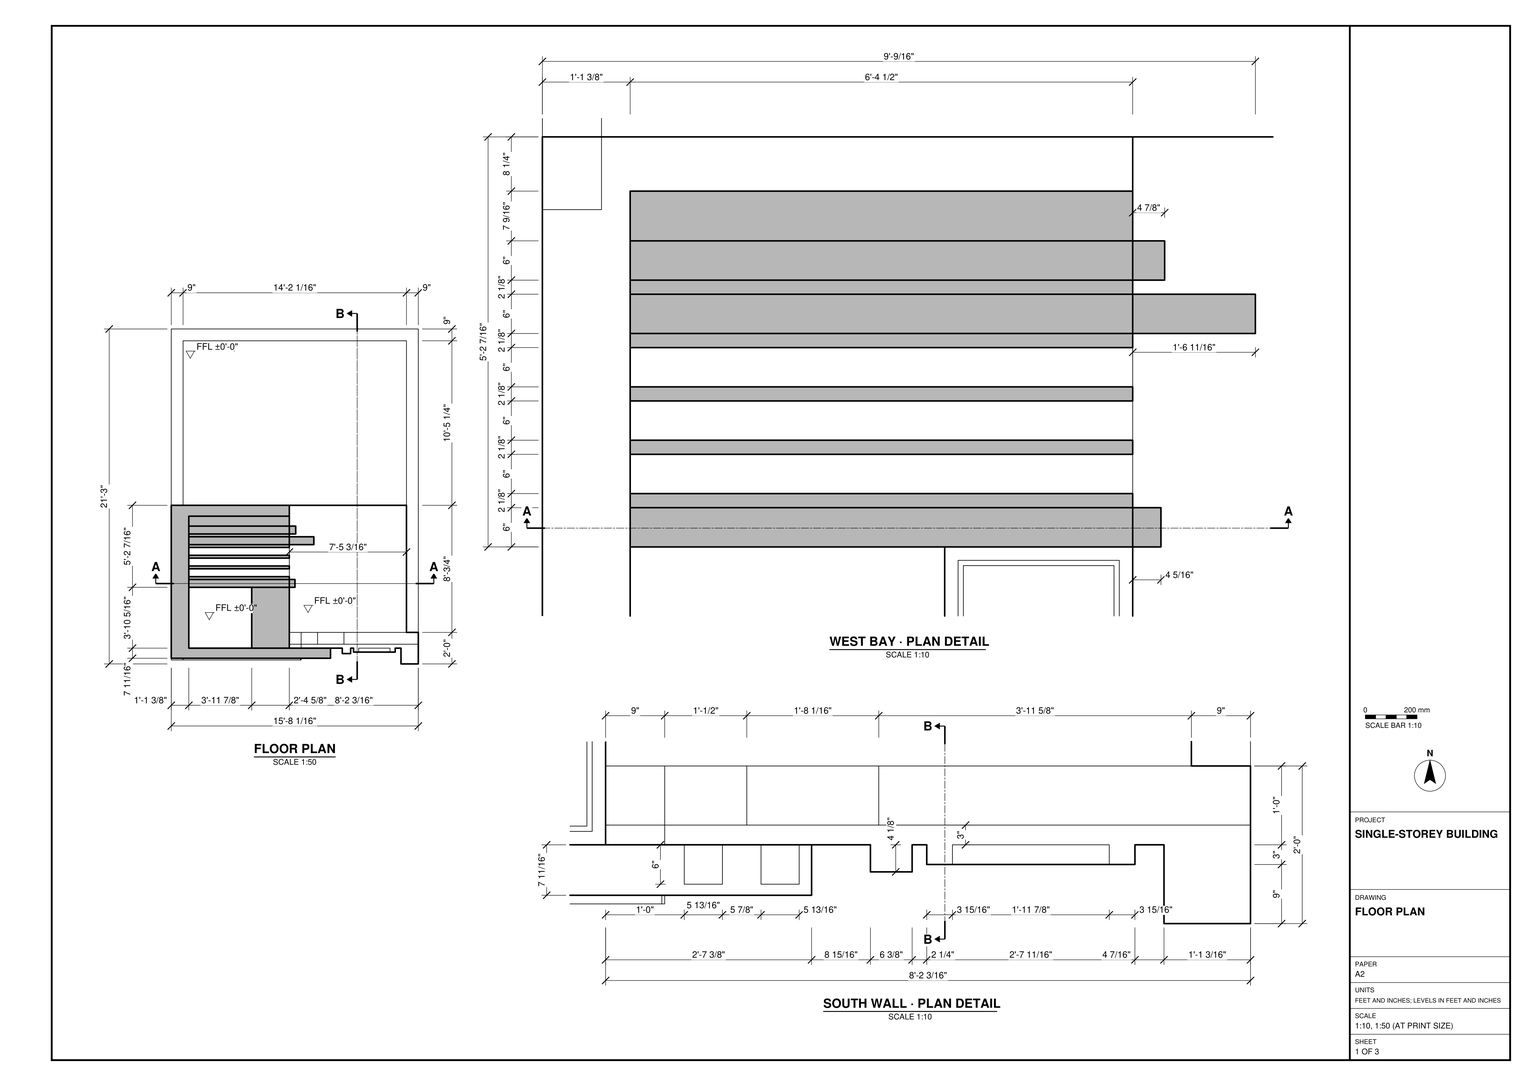
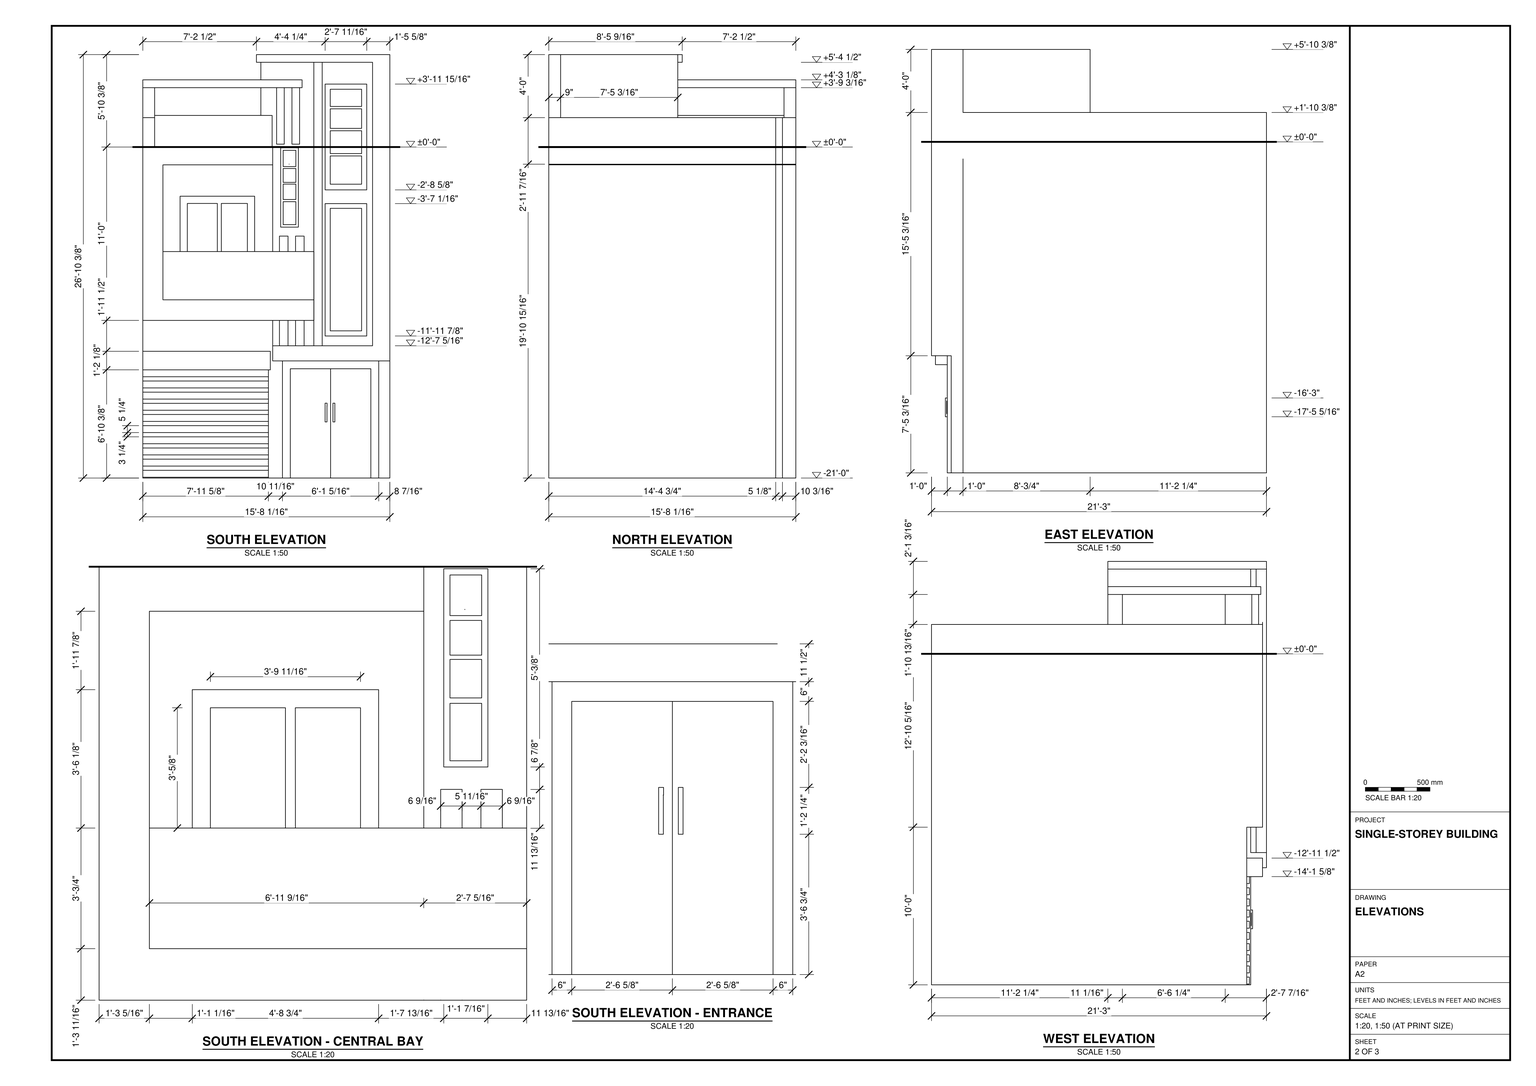
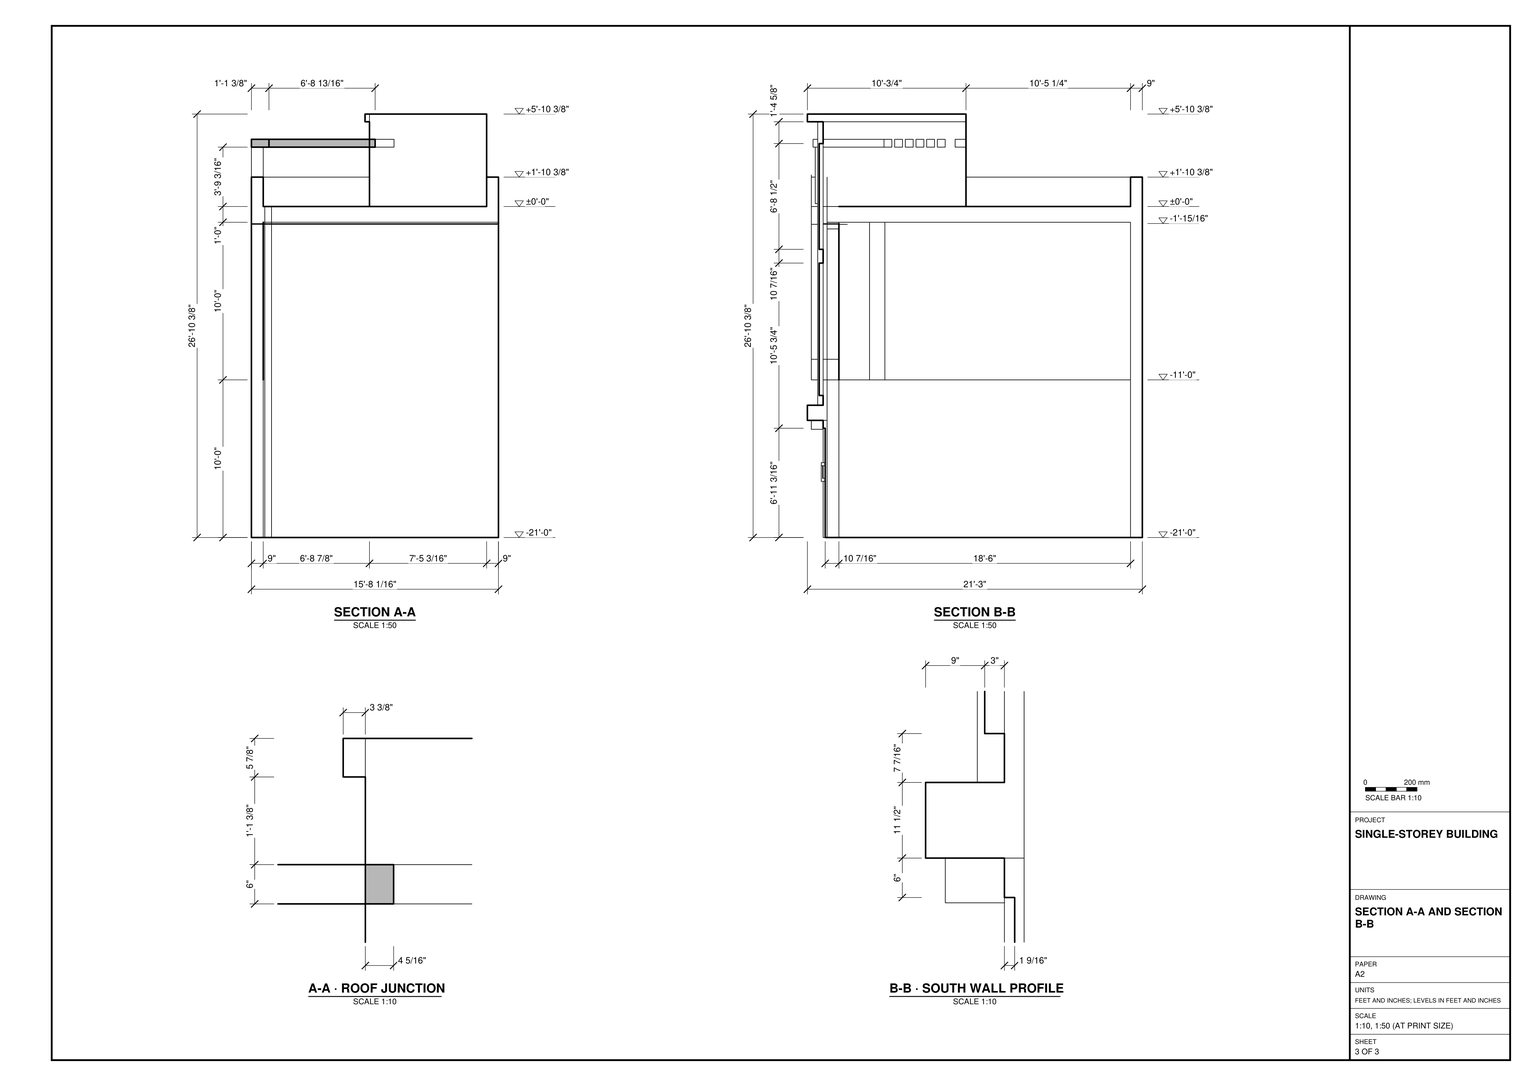
Build the single-storey building in SketchUp from task_files/diagram_01.pdf. Work in feet and inches. Set out the rectangular shell at 15'-8 1/16" east to west and 21'-3" north to south, with an overall height of 26'-10 3/8". Use the finished level marked ±0'-0" as the drawing datum. Follow the sections for the position of the roof slab relative to this datum and the base of the walls.

Use the wall thicknesses shown in plan. On the south face, place the horizontally slatted bay to the left of the double entrance doors. Above them, model the recessed central bay, its solid lower panel, the framed openings and the tall panelled strip on the right. Use the south wall plan and section details to give the ledges and recesses their drawn depths. At the roof, distinguish the low rear parapet from the raised front framing. Lay out the parallel members over the west bay with the different end projections shown in plan.

Keep walls, slabs, roof elements and any joinery pieces in separate groups or components, and use components for repeated parts. Any decor or loose items shown may be suitable library components. Save one SketchUp model as output_files/single_storey_building_with_a_stepped_south_facade.skp.

# SketchUp Ruby script. Lengths in inches.
U = 1.inch
M = Sketchup.active_model
def pt(a) = Geom::Point3d.new(a.map { |v| v * U })
def face(e, loops, mat)
  f = e.add_face(loops[0].map { |a| pt(a) })
  loops[1..].each { |l| e.add_face(l.map { |a| pt(a) }).erase! }
  f.material = f.back_material = mat if mat
  f
end
# faces: each face lists its corners as indices into pts; further lists are holes
def faces(e, pts, list, mat = nil) = list.each { |f| face(e, (f[0].is_a?(Array) ? f : [f]).map { |l| l.map { |i| pts[i] } }, mat) }
# xy, xz, yz: faces in a plane at the given z, y or x. An outline is a flat list of corners, or four numbers for a rectangle; further outlines are holes
def ring(l) = l.size == 4 ? [[l[0], l[1]], [l[2], l[1]], [l[2], l[3]], [l[0], l[3]]] : l.each_slice(2).to_a
def flat(e, list, mat, &to3) = list.each { |f| face(e, (f[0].is_a?(Array) ? f : [f]).map { |l| ring(l).map { |u, v| to3.(u, v) } }, mat) }
def xy(e, z, list, mat = nil) = flat(e, list, mat) { |x, y| [x, y, z] }
def xz(e, y, list, mat = nil) = flat(e, list, mat) { |x, z| [x, y, z] }
def yz(e, x, list, mat = nil) = flat(e, list, mat) { |y, z| [x, y, z] }
def lines(e, pts, list) = list.each { |a, b| e.add_line(pt(pts[a]), pt(pts[b])) }
# prism: a flat outline (further loops are holes) pulled along v
def prism(e, loops, v, mat = nil)
  f = face(e, loops, mat); d = Geom::Vector3d.new(v.map { |x| x * U })
  f.pushpull(f.normal.samedirection?(d) ? d.length : -d.length)
end
def box(e, o, s, mat = nil) = prism(e, [[o, [o[0] + s[0], o[1], o[2]], [o[0] + s[0], o[1] + s[1], o[2]], [o[0], o[1] + s[1], o[2]]]], [0, 0, s[2]], mat)
def at(x, y, z, deg = 0) = Geom::Transformation.translation(pt([x, y, z])) * Geom::Transformation.rotation(ORIGIN, Z_AXIS, deg.degrees)
def axes(o, x, y, z) = Geom::Transformation.new([*x, 0, *y, 0, *z, 0, *pt(o).to_a, 1])
def part(name) = M.definitions.add(name)
# library, detail: a bought-in or finely detailed component or shape, given as its bounding box
def library(name, o, s) = part(name).tap { |d| box(d.entities, o, s) }
def detail(e, o, s) = box(e.add_group.entities, o, s)
def put(e, d, t, mat = nil) = e.add_instance(d, t).tap { |i| i.material = mat if mat }
def group(e, t, mat = nil) = e.add_group.tap { |g| g.transformation = t; g.material = mat if mat }.entities
root = M.entities
M.materials.add("[0036_BurlyWood]").color = [145, 120, 88]
M.materials.add("[0135_DarkGray]").color = [81, 81, 81]
M.materials.add("[Blinds Roman Hobbled Blue]").color = [81, 82, 87]
M.materials.add("[Color B08]").color = [102, 25, 0]
M.materials.add("[Color C05]").color = [216, 107, 0]
M.materials.add("[Color M09]").color = [0, 0, 0]
M.materials.add("[Concrete Scored Jointless]").color = [15, 14, 13]
M.materials.add("[Translucent Glass Blue]").color = [100, 149, 237]
M.materials["[Translucent Glass Blue]"].alpha = 0.5
M.materials.add("[Translucent Glass Gray]").color = [117, 117, 117]
M.materials["[Translucent Glass Gray]"].alpha = 0.5
M.materials.add("[Translucent Glass Gray]1").color = [99, 99, 99]
M.materials["[Translucent Glass Gray]1"].alpha = 0.5
M.materials.add("[Wood Bamboo]").color = [177, 105, 43]
M.materials.add("[Wood Veneer 01]").color = [120, 70, 37]
xy(root,0,[[106.29,12,106.29,15,0,15,0,255,188.0625,255,188.0625,15,179.6,15,179.6,12,173.6,12,173.6,13.5625,112.29,13.5625,112.29,12]])
xy(root,0.62,[[0,13,95.6,15]],"[Blinds Roman Hobbled Blue]")
xy(root,5.88,[[0,13,95.6,15]],"[Blinds Roman Hobbled Blue]")
xy(root,9.12,[[0,13,95.6,15]],"[Blinds Roman Hobbled Blue]")
xy(root,14.38,[[0,13,95.6,15]],"[Blinds Roman Hobbled Blue]")
xy(root,17.62,[[0,13,95.6,15]],"[Blinds Roman Hobbled Blue]")
xy(root,22.88,[[0,13,95.6,15]],"[Blinds Roman Hobbled Blue]")
xy(root,26.12,[[0,13,95.6,15]],"[Blinds Roman Hobbled Blue]")
xy(root,31.38,[[0,13,95.6,15]],"[Blinds Roman Hobbled Blue]")
xy(root,34.62,[[0,13,95.6,15]],"[Blinds Roman Hobbled Blue]")
xy(root,39.88,[[0,13,95.6,15]],"[Blinds Roman Hobbled Blue]")
xy(root,42.73,[[138.76,10.5625,140.19,13.5625],[144.76,10.5625,146.19,13.5625]],"[Concrete Scored Jointless]")
xy(root,43.12,[[0,13,95.6,15]],"[Blinds Roman Hobbled Blue]")
xy(root,45.05,[[138.76,11.5625,140.19,13.5625],[144.76,11.5625,146.19,13.5625]])
xy(root,48.38,[[0,13,95.6,15]],"[Blinds Roman Hobbled Blue]")
xy(root,51.62,[[0,13,95.6,15]],"[Blinds Roman Hobbled Blue]")
xy(root,54.67,[[140.19,10.5625,140.26,11.5625]])
xy(root,54.67,[[138.76,11.5625,140.26,13.5625],[144.76,11.5625,146.19,13.5625]],"[Concrete Scored Jointless]")
xy(root,56.88,[[0,13,95.6,15]],"[Blinds Roman Hobbled Blue]")
xy(root,56.99,[[138.76,10.5625,140.26,13.5625],[144.76,10.5625,146.19,13.5625]])
xy(root,60.12,[[0,13,95.6,15]],"[Blinds Roman Hobbled Blue]")
xy(root,65.38,[[0,13,95.6,15]],"[Blinds Roman Hobbled Blue]")
xy(root,68.62,[[0,13,95.6,15]],"[Blinds Roman Hobbled Blue]")
xy(root,73.88,[[0,13,95.6,15]],"[Blinds Roman Hobbled Blue]")
xy(root,77.12,[[0,13,95.6,15]],"[Blinds Roman Hobbled Blue]")
xy(root,82.38,[[0,13,95.6,15]])
xy(root,82.38,[[0,3,0,13,95.6,13,95.6,15,97.0625,15,97.0625,3]],"[0135_DarkGray]")
xy(root,83.1875,[[112.29,12,113.71,13.5625],[113.71,12,130.28,13.5625],[130.28,12,173.6,13.5625]],"[Concrete Scored Jointless]")
xy(root,89.1875,[[98.875,0,98.875,15,106.29,15,106.29,12,179.6,12,179.6,15,188.0625,15,188.0625,0],[106.29,12,113.71,15],[113.71,12,130.28,15]])
xy(root,96.5,[[0,3,97.0625,15]],"[0135_DarkGray]")
xy(root,100.7,[[104.02,7.875,110.53,12],[116.27,7.875,122.78,12]])
xy(root,100.7,[[98.875,0,174.89,0,174.89,12,136.55,12,136.55,7.875,130.2,7.875,130.2,12,122.78,12,122.78,7.875,116.27,7.875,116.27,12,110.53,12,110.53,7.875,104.02,7.875,104.02,12,98.875,12]],"[0036_BurlyWood]")
xy(root,108.15,[[138.77,9,170.47,12]])
xy(root,112.06,[[142.68,9,166.56,12]],"[Wood Veneer 01]")
xy(root,120,[[0,3,0,15,113.71,15,113.71,12,116.27,12,116.27,7.875,122.78,7.875,122.78,12,130.25,12,130.25,3],[116.27,7.875,122.78,12],[113.71,12,130.25,15],[130.25,12,130.28,15],[9,15,15.3125,24],
  [130.25,15,130.28,24],[130.28,15,131.46,24],[28.37,21,33.88,24],[56.74,21,59.8125,24],[79.6,21,85.12,24],
  [9,24,131.46,47.3125]])
xy(root,120,[[15.3125,15,130.25,15,130.25,24,85.12,24,85.12,21,79.6,21,79.6,24,59.8125,24,59.8125,21,56.74,21,56.74,24,33.88,24,33.88,21,28.37,21,28.37,24,15.3125,24]],"[0036_BurlyWood]")
xy(root,135.6875,[[98.875,15,130.25,24]])
xy(root,135.6875,[[15.3125,3,130.25,15]],"[0036_BurlyWood]")
xy(root,184.19,[[104.02,7.875,110.53,12],[116.27,7.875,122.78,12]],"[Color C05]")
xy(root,191.01,[[104.95,9,118.39,12]],"[Wood Veneer 01]")
xy(root,192.91,[[106.85,9,116.5,12]],"[Wood Veneer 01]")
xy(root,205.33,[[142.68,9,166.56,12]],"[Wood Veneer 01]")
xy(root,208.92,[[138.77,9,170.47,12]],"[Wood Veneer 01]")
xy(root,209.05,[[33.88,21,56.74,24],[59.75,21,79.6,24]],"[Color M09]")
xy(root,210.4,[[106.85,9,116.5,12]],"[Wood Veneer 01]")
xy(root,212.05,[[106.85,9,116.5,12]],"[Wood Veneer 01]")
xy(root,214.5625,[[28.37,21,85.12,24]],"[Color M09]")
xy(root,219.38,[[138.77,9,170.47,12]],"[Wood Veneer 01]")
xy(root,223.71,[[142.68,9,166.56,12]],"[Wood Veneer 01]")
xy(root,223.78,[[106.85,9,116.5,12]],"[Wood Veneer 01]")
xy(root,225.08,[[106.85,9,116.5,12]],"[Wood Veneer 01]")
xy(root,234.9375,[[111.375,15,130.28,24]])
xy(root,235.65,[[106.85,9,116.5,12]],"[Wood Veneer 01]")
xy(root,237.12,[[106.85,9,116.5,12]],"[Wood Veneer 01]")
xy(root,238.4375,[[15.3125,3,98.875,30.4375],[98.875,15,111.375,24]])
xy(root,240,[[9,15,15.3125,24]])
xy(root,245.21,[[142.68,9,166.56,12]],"[Wood Veneer 01]")
xy(root,247.01,[[142.68,9,166.56,12]],"[Wood Veneer 01]")
xy(root,249.5,[[106.85,9,116.5,12]],"[Wood Veneer 01]")
xy(root,251.39,[[104.95,9,118.39,12]],"[Wood Veneer 01]")
xy(root,252,[[9,3,98.4375,12],[98.4375,3,98.875,12],[9,12,89.875,12,89.875,120.75,179.0625,120.75,179.0625,246,9,246],[89.875,24,179.0625,120.75]])
xy(root,254.18,[[101.85,6,107.66,12],[113.54,6,119.35,12]],"[Color C05]")
xy(root,264.4,[[142.68,9,166.56,12]],"[Wood Veneer 01]")
xy(root,266.2,[[142.68,9,166.56,12]],"[Wood Veneer 01]")
xy(root,274.375,[[0,11.16,9,14.35],[0,14.35,9,31.41],[179.0625,24,188.0625,24,188.0625,255,0,255,0,120.75,9,120.75,9,246,179.0625,246],[0,31.41,9,109.67],[0,109.67,9,120.75]])
xy(root,274.375,[[0,3,9,11.16]],"[0036_BurlyWood]")
xy(root,281.09,[[142.68,9,166.56,12]],"[Wood Veneer 01]")
xy(root,282.89,[[142.68,9,166.56,12]],"[Wood Veneer 01]")
xy(root,296,[[142.68,9,166.56,12]],"[Wood Veneer 01]")
xy(root,297.18,[[0,4.3125,0,109.67,9,109.67,9,120.75,89.875,120.75,89.875,112.49,13.37,112.49,13.37,12,101.85,12,101.85,6,107.66,6,107.66,12,113.54,12,113.54,6,119.35,6,119.35,12,121.24,12,121.24,4.3125],[101.85,6,107.66,12],[113.54,6,119.35,12],[[63.29,14.04,87.83,56.27],[64.09,14.84,87.03,55.47]],[13.37,58.3125,94.18,64.29],
  [13.37,66.4375,89.875,72.42],[13.37,74.5625,89.875,80.54],[13.37,82.6875,89.875,88.67],[13.37,90.8125,108.55,96.79],[13.37,98.9375,94.74,104.92],
  [0,109.67,9,120.75]])
xy(root,297.18,[[[61.25,12,89.875,58.3125],[63.29,14.04,87.83,56.27]],[64.09,14.84,87.03,55.47]],"[Color B08]")
xy(root,297.1875,[[0,11.16,9,14.35],[0,14.35,9,31.41]])
xy(root,299.91,[[138.77,9,170.47,12]],"[Wood Veneer 01]")
xy(root,303.16,[[0,4.3125,121.24,4.3125,121.24,12,13.37,12,13.37,112.49,89.875,112.49,89.875,120.75,0,120.75],[61.25,12,89.875,58.3125],[13.37,58.3125,94.18,64.29],[13.37,66.4375,89.875,72.42],[13.37,74.5625,89.875,80.54],
  [13.37,82.6875,89.875,88.67],[13.37,90.8125,108.55,96.79],[13.37,98.9375,94.74,104.92]])
xy(root,316.51,[[86.5,0,86.5,120.75,89.875,120.75,89.875,12,130.2,12,130.2,7.875,136.55,7.875,136.55,12,174.89,12,174.89,0]],"[0036_BurlyWood]")
xy(root,322.375,[[86.5,0,188.0625,0,188.0625,24,179.0625,24,179.0625,120.75,86.5,120.75]],"[0036_BurlyWood]")
xz(root,0,[[98.875,89.1875,188.0625,89.1875,188.0625,322.375,86.5,322.375,86.5,316.51,174.89,316.51,174.89,100.7,98.875,100.7]],"[0036_BurlyWood]")
xz(root,3,[[0,120,130.25,120,130.25,135.6875,15.3125,135.6875,15.3125,238.4375,98.875,238.4375,98.875,252,9,252,9,274.375,0,274.375]],"[0036_BurlyWood]")
xz(root,3,[[0,82.38,97.0625,96.5]],"[0135_DarkGray]")
xz(root,3,[[15.3125,135.6875,130.25,172.42],[9,252,98.4375,276.0625]],"[Translucent Glass Gray]")
xz(root,4.3125,[[0,297.18,121.24,303.16]])
xz(root,6,[[101.85,254.18,107.66,297.18],[113.54,254.18,119.35,297.18]],"[Color C05]")
xz(root,7.875,[[104.02,100.7,110.53,184.19],[116.27,100.7,122.78,120],[130.2,100.7,136.55,316.51],[116.27,120,122.78,184.19]],"[Color C05]")
xz(root,9,[[[138.77,108.15,170.47,208.92],[142.68,112.06,166.56,205.33]],[[104.95,191.01,118.39,251.39],[106.85,192.91,116.5,210.4],[106.85,237.12,116.5,249.5],[106.85,212.05,116.5,223.78],[106.85,225.08,116.5,235.65]],[[138.77,219.38,170.47,299.91],[142.68,223.71,166.56,245.21],[142.68,247.01,166.56,264.4],[142.68,266.2,166.56,281.09],[142.68,282.89,166.56,296]]],"[Wood Veneer 01]")
xz(root,10.5625,[[138.76,42.73,140.19,42.73,140.19,54.67,140.26,54.67,140.26,56.99,138.76,56.99],[144.76,42.73,146.19,56.99]],"[Concrete Scored Jointless]")
xz(root,11.16,[[0,274.375,9,297.1875]])
xz(root,11.5625,[[138.76,45.05,140.19,54.67],[144.76,45.05,146.19,54.67]])
xz(root,12,[[104.02,100.7,110.53,184.19],[116.27,100.7,122.78,120],[116.27,120,122.78,184.19],[101.85,254.18,107.66,272.8],[113.54,254.18,119.35,272.8],
  [101.85,272.8,107.66,297.18],[113.54,272.8,119.35,297.18],[13.37,297.18,61.25,303.16],[61.25,297.18,89.875,303.16],[89.875,297.18,121.24,303.16]])
xz(root,12,[[[98.875,100.7,104.02,100.7,104.02,184.19,110.53,184.19,110.53,100.7,116.27,100.7,116.27,184.19,122.78,184.19,122.78,120,130.2,120,130.2,316.51,89.875,316.51,89.875,303.16,121.24,303.16,121.24,297.18,119.35,297.18,119.35,254.18,113.54,254.18,113.54,297.18,107.66,297.18,107.66,254.18,101.85,254.18,101.85,297.18,89.875,297.18,89.875,252,98.875,252],[104.95,191.01,118.39,251.39]],[122.78,100.7,130.2,120],[[136.55,100.7,174.89,316.51],[138.77,108.15,170.47,208.92],[138.77,219.38,170.47,299.91]]],"[0036_BurlyWood]")
xz(root,12,[[106.29,0,112.29,0,112.29,83.1875,173.6,83.1875,173.6,0,179.6,0,179.6,89.1875,106.29,89.1875]],"[Concrete Scored Jointless]")
xz(root,12,[[142.68,112.06,166.56,205.33],[142.68,223.71,166.56,245.21],[142.68,247.01,166.56,264.4],[142.68,266.2,166.56,281.09],[142.68,282.89,166.56,296]],"[Translucent Glass Gray]1")
xz(root,12,[[106.85,192.91,116.5,210.4],[106.85,212.05,116.5,223.78],[106.85,225.08,116.5,235.65],[106.85,237.12,116.5,249.5]],"[Wood Bamboo]")
xz(root,13,[[0,0.62,95.6,5.88],[0,9.12,95.6,14.38],[0,17.62,95.6,22.88],[0,26.12,95.6,31.38],[0,34.62,95.6,39.88],
  [0,43.12,95.6,48.38],[0,51.62,95.6,56.88],[0,60.12,95.6,65.38],[0,68.62,95.6,73.88],[0,77.12,95.6,82.38]],"[Blinds Roman Hobbled Blue]")
xz(root,13.5625,[[[112.29,0,142.95,83.1875],[138.76,54.67,140.26,56.99],[138.76,42.73,140.19,45.05]],[[142.95,0,173.6,83.1875],[144.76,54.67,146.19,56.99],[144.76,42.73,146.19,45.05]]],"[Concrete Scored Jointless]")
xz(root,15,[[0,0,95.6,0.62],[0,0.62,95.6,5.88],[0,9.12,95.6,14.38],[0,17.62,95.6,22.88],[0,26.12,95.6,31.38],
  [0,34.62,95.6,39.88],[0,43.12,95.6,48.38],[0,51.62,95.6,56.88],[0,60.12,95.6,65.38],[0,68.62,95.6,73.88],
  [0,77.12,95.6,82.38],[0,82.38,97.0625,96.5],[98.875,89.1875,113.71,102.3125],[113.71,89.1875,130.28,102.3125],[98.875,102.3125,113.71,120],
  [113.71,102.3125,130.28,113.3125],[113.71,113.3125,130.28,120],[98.875,120,130.25,135.6875],[130.28,120,131.46,234.9375],[111.375,234.9375,130.28,238.4375],
  [130.28,234.9375,131.46,238.4375],[98.875,238.4375,111.375,239.04],[111.375,238.4375,130.28,238.9375],[130.28,238.4375,131.46,238.9375],[111.375,238.9375,130.28,239.04],
  [130.28,238.9375,131.46,239.04],[111.375,239.04,130.28,240],[130.28,239.04,131.46,240]])
xz(root,15,[[95.6,0,106.29,0,106.29,89.1875,98.875,89.1875,98.875,120,0,120,0,96.5,97.0625,96.5,97.0625,82.38,95.6,82.38],[179.6,0,188.0625,89.1875],[15.3125,120,98.875,135.6875]],"[0036_BurlyWood]")
xz(root,15,[[0,5.88,95.6,9.12],[0,14.38,95.6,17.62],[0,22.88,95.6,26.12],[0,31.38,95.6,34.62],[0,39.88,95.6,43.12],
  [0,48.38,95.6,51.62],[0,56.88,95.6,60.12],[0,65.38,95.6,68.62],[0,73.88,95.6,77.12]],"[Blinds Roman Hobbled Blue]")
xz(root,21,[[28.37,120,33.88,120,33.88,209.05,56.74,209.05,56.74,120,59.8125,120,59.75,209.05,79.6,209.05,79.6,120,85.12,120,85.12,214.5625,28.37,214.5625]],"[Color M09]")
xz(root,24,[[9,120,15.3125,240],[98.875,234.9375,111.375,238.4375],[179.0625,274.375,188.0625,322.375]])
xz(root,24,[[15.3125,120,28.37,120,28.37,214.5625,85.12,214.5625,85.12,120,130.25,120,130.25,135.6875,98.875,135.6875,98.875,238.4375,111.375,238.4375,111.375,234.9375,130.28,234.9375,130.28,120,188.0625,120,188.0625,239.04,15.3125,239.04]],"[0036_BurlyWood]")
xz(root,24,[[33.88,120,56.74,209.05],[59.8125,120,79.6,120,79.6,209.05,59.75,209.05]],"[Translucent Glass Blue]")
xz(root,31.41,[[0,274.375,9,297.1875]])
xz(root,58.3125,[[13.37,297.18,61.25,303.16],[61.25,297.18,89.875,303.16],[89.875,297.18,94.18,303.16]])
xz(root,64.29,[[13.37,297.18,94.18,303.16]])
xz(root,66.4375,[[13.37,297.18,89.875,303.16]])
xz(root,72.42,[[13.37,297.18,89.875,303.16]])
xz(root,74.5625,[[13.37,297.18,89.875,303.16]])
xz(root,80.54,[[13.37,297.18,89.875,303.16]])
xz(root,82.6875,[[13.37,297.18,89.875,303.16]])
xz(root,88.67,[[13.37,297.18,89.875,303.16]])
xz(root,90.8125,[[13.37,297.18,108.55,303.16]])
xz(root,96.79,[[13.37,297.18,108.55,303.16]])
xz(root,98.9375,[[13.37,297.18,94.74,303.16]])
xz(root,104.92,[[13.37,297.18,94.74,303.16]])
xz(root,109.67,[[0,274.375,9,297.18]])
xz(root,112.49,[[13.37,297.18,89.875,303.16]])
xz(root,120.75,[[89.875,252,179.0625,322.375],[0,274.375,9,297.18],[0,297.18,89.875,303.16],[86.5,316.51,89.875,322.375]])
xz(root,246,[[9,252,179.0625,274.375]])
xz(root,255,[[0,0,10.1875,238.4375],[10.1875,0,15.3125,238.4375],[15.3125,0,188.0625,238.4375],[0,238.4375,10.1875,238.9375],[10.1875,238.4375,15.3125,238.9375],
  [15.3125,238.4375,188.0625,238.9375],[0,238.9375,10.1875,274.375],[10.1875,238.9375,15.3125,274.375],[15.3125,238.9375,188.0625,274.375]])
yz(root,0,[[15,0,15,120,3,120,3,274.375,255,274.375,255,0],[11.16,274.375,31.41,297.18],[109.67,274.375,120.75,297.18],[4.3125,297.18,4.3125,303.16,120.75,303.16,120.75,297.18,31.41,297.18,31.41,297.1875,11.16,297.1875,11.16,297.18],[11.16,297.18,14.35,297.1875],
  [14.35,297.18,31.41,297.1875]])
yz(root,0,[[3,82.38,15,96.5]],"[0135_DarkGray]")
yz(root,0,[[13,0.62,15,5.88],[13,9.12,15,14.38],[13,17.62,15,22.88],[13,26.12,15,31.38],[13,34.62,15,39.88],
  [13,43.12,15,48.38],[13,51.62,15,56.88],[13,60.12,15,65.38],[13,68.62,15,73.88],[13,77.12,15,82.38]],"[Blinds Roman Hobbled Blue]")
yz(root,9,[[15,120,24,240],[24,120,47.3125,240],[47.3125,120,59,240],[47.3125,120,59,240],[47.3125,120,59,240],
  [59,120,246,240],[3,252,12,274.375],[12,252,246,274.375],[11.16,274.375,14.35,297.1875],[14.35,274.375,31.41,297.1875],
  [109.67,274.375,120.75,297.18]])
yz(root,13.37,[[12,297.18,58.3125,303.16],[58.3125,297.18,64.29,303.16],[64.29,297.18,66.4375,303.16],[66.4375,297.18,72.42,303.16],[72.42,297.18,74.5625,303.16],
  [74.5625,297.18,80.54,303.16],[80.54,297.18,82.6875,303.16],[82.6875,297.18,88.67,303.16],[88.67,297.18,90.8125,303.16],[90.8125,297.18,96.79,303.16],
  [96.79,297.18,98.9375,303.16],[98.9375,297.18,104.92,303.16],[104.92,297.18,112.49,303.16]])
yz(root,15.3125,[[15,239.04,24,240]])
yz(root,15.3125,[[15,120,24,120,24,238.4375,3,238.4375,3,135.6875,15,135.6875]],"[0036_BurlyWood]")
yz(root,28.37,[[21,120,24,214.5625]],"[Color M09]")
yz(root,33.88,[[21,120,24,209.05]],"[Color M09]")
yz(root,56.74,[[21,120,24,209.05]],"[Color M09]")
yz(root,61.25,[[12,297.18,58.3125,303.16]])
yz(root,79.6,[[21,120,24,209.05]],"[Color M09]")
yz(root,85.12,[[21,120,24,214.5625]],"[Color M09]")
yz(root,86.5,[[0,316.51,120.75,322.375]],"[0036_BurlyWood]")
yz(root,89.875,[[12,297.18,58.3125,303.16],[112.49,297.18,120.75,303.16]])
yz(root,89.875,[[[12,252,12,297.18,58.3125,297.18,58.3125,303.16,12,303.16,12,316.51,120.75,316.51,120.75,303.16,112.49,303.16,112.49,297.18,120.75,297.18,120.75,252],[82.6875,297.18,88.67,303.16],[74.5625,297.18,80.54,303.16],[66.4375,297.18,72.42,303.16]]],"[0036_BurlyWood]")
yz(root,94.18,[[58.3125,297.18,64.29,303.16]])
yz(root,94.74,[[98.9375,297.18,104.92,303.16]])
yz(root,95.6,[[13,0.62,15,5.88],[13,9.12,15,14.38],[13,17.62,15,22.88],[13,26.12,15,31.38],[13,34.62,15,39.88],
  [13,43.12,15,48.38],[13,51.62,15,56.88],[13,60.12,15,65.38],[13,68.62,15,73.88],[13,77.12,15,82.38]],"[Blinds Roman Hobbled Blue]")
yz(root,97.0625,[[3,82.38,15,96.5]],"[0135_DarkGray]")
yz(root,98.4375,[[3,252,12,274.375]],"[Translucent Glass Gray]")
yz(root,98.875,[[12,238.4375,15,239.04]])
yz(root,98.875,[[0,89.1875,0,100.7,12,100.7,12,238.4375,24,238.4375,24,135.6875,15,135.6875,15,89.1875],[3,238.4375,12,252]],"[0036_BurlyWood]")
yz(root,101.85,[[6,254.18,12,297.18]],"[Color C05]")
yz(root,104.02,[[7.875,100.7,12,184.19]],"[Color C05]")
yz(root,104.95,[[9,191.01,12,251.39]],"[Wood Veneer 01]")
yz(root,106.29,[[12,0,15,89.1875]])
yz(root,106.85,[[9,192.91,12,210.4],[9,212.05,12,223.78],[9,225.08,12,235.65],[9,237.12,12,249.5]],"[Wood Veneer 01]")
yz(root,107.66,[[6,254.18,12,297.18]],"[Color C05]")
yz(root,108.55,[[90.8125,297.18,96.79,303.16]])
yz(root,110.53,[[7.875,100.7,12,184.19]],"[Color C05]")
yz(root,111.375,[[15,234.9375,24,238.4375]])
yz(root,112.29,[[12,0,13.5625,83.1875]],"[Concrete Scored Jointless]")
yz(root,113.54,[[6,254.18,12,297.18]],"[Color C05]")
yz(root,116.27,[[7.875,100.7,12,120],[7.875,120,12,184.19]],"[Color C05]")
yz(root,116.5,[[9,192.91,12,210.4],[9,212.05,12,223.78],[9,225.08,12,235.65],[9,237.12,12,249.5]],"[Wood Veneer 01]")
yz(root,118.39,[[9,191.01,12,251.39]],"[Wood Veneer 01]")
yz(root,119.35,[[6,254.18,12,297.18]],"[Color C05]")
yz(root,121.24,[[4.3125,297.18,12,303.16]])
yz(root,122.78,[[7.875,100.7,12,120],[7.875,120,12,184.19]],"[Color C05]")
yz(root,130.2,[[7.875,100.7,12,316.51]],"[Color C05]")
yz(root,130.25,[[15,120,24,135.6875]])
yz(root,130.25,[[3,120,15,135.6875]],"[0036_BurlyWood]")
yz(root,130.28,[[15,120,24,234.9375]])
yz(root,136.55,[[7.875,100.7,12,316.51]],"[Color C05]")
yz(root,138.76,[[10.5625,42.73,10.5625,56.99,13.5625,56.99,13.5625,54.67,11.5625,54.67,11.5625,45.05,13.5625,45.05,13.5625,42.73]],"[Concrete Scored Jointless]")
yz(root,138.77,[[9,108.15,12,208.92],[9,219.38,12,299.91]],"[Wood Veneer 01]")
yz(root,140.19,[[10.5625,42.73,13.5625,42.73,13.5625,45.05,11.5625,45.05,11.5625,54.67,10.5625,54.67]],"[Concrete Scored Jointless]")
yz(root,140.26,[[10.5625,54.67,13.5625,56.99]],"[Concrete Scored Jointless]")
yz(root,142.68,[[9,112.06,12,205.33],[9,223.71,12,245.21],[9,247.01,12,264.4],[9,266.2,12,281.09],[9,282.89,12,296]],"[Wood Veneer 01]")
yz(root,144.76,[[10.5625,42.73,10.5625,56.99,13.5625,56.99,13.5625,54.67,11.5625,54.67,11.5625,45.05,13.5625,45.05,13.5625,42.73]],"[Concrete Scored Jointless]")
yz(root,146.19,[[10.5625,42.73,13.5625,42.73,13.5625,45.05,11.5625,45.05,11.5625,54.67,13.5625,54.67,13.5625,56.99,10.5625,56.99]],"[Concrete Scored Jointless]")
yz(root,166.56,[[9,112.06,12,205.33],[9,223.71,12,245.21],[9,247.01,12,264.4],[9,266.2,12,281.09],[9,282.89,12,296]],"[Wood Veneer 01]")
yz(root,170.47,[[9,108.15,12,208.92],[9,219.38,12,299.91]],"[Wood Veneer 01]")
yz(root,173.6,[[12,0,13.5625,83.1875]],"[Concrete Scored Jointless]")
yz(root,174.89,[[0,100.7,12,316.51]],"[0036_BurlyWood]")
yz(root,179.0625,[[24,252,120.75,274.375],[120.75,252,246,274.375],[24,274.375,120.75,322.375]])
yz(root,179.6,[[12,0,15,89.1875]])
yz(root,188.0625,[[15,0,24,0,24,120,24,0,255,0,255,274.375,24,274.375,24,322.375,0,322.375,0,89.1875,15,89.1875]],"[0036_BurlyWood]")
p = [[59.8125,24,120],[59.75,24,209.05],[59.75,21,209.05],[59.8125,21,120],[131.46,47.3125,240],[131.46,47.3125,120],
  [188.0625,15,120],[131.46,15,120],[9,59,120],[188.0625,59,120],[9,246,240],[188.0625,246,240],
  [131.46,24,240],[131.46,15,240],[9,47.3125,240],[98.875,15,234.9375],[111.375,15,234.9375],[9,246,0],
  [9,246,120],[9,24,0],[9,24,120],[9,15,234.9375],[15.3125,15,234.9375],[15.3125,15,240],
  [111.375,15,240],[111.375,3,239.04],[111.375,3,238.9375],[131.46,15,238.4375],[188.0625,15,238.4375],[131.46,15,274.375],
  [79.6,24,120],[79.6,24,119.77],[15.3125,15,135.6875],[98.875,14.97,135.6875],[174.89,12,100.7],[188.0625,15,100.7]]
faces(root,p,[[0,1,2,3]],"[Color M09]")
lines(root,p,[[4,5],[6,7],[8,9],[10,11],[12,13],[14,4],[15,16],[17,18],[19,20],[21,22],[23,24],[25,26],
  [27,28],[29,13],[30,31],[32,33],[34,35]])
